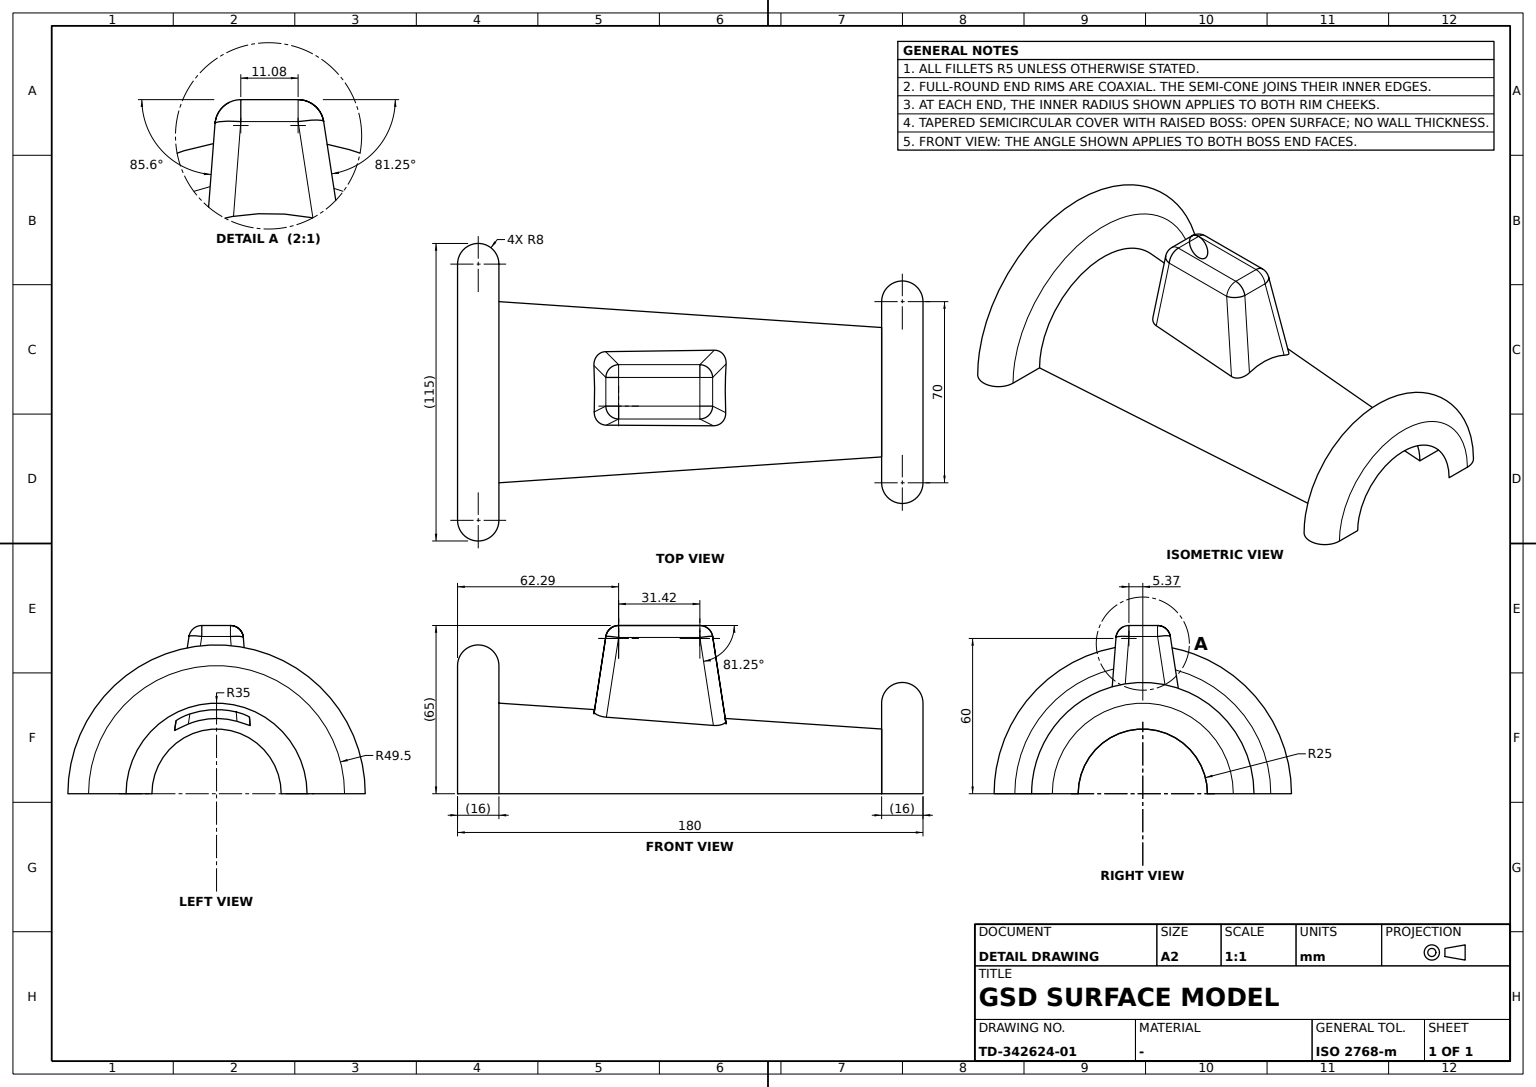
ISO-10303-21;
HEADER;
FILE_DESCRIPTION((''),'2;1');
FILE_NAME('','',(''),(''),'','','');
FILE_SCHEMA(('AUTOMOTIVE_DESIGN'));
ENDSEC;
DATA;
#1=CIRCLE('',#302,4.999999999999998224);
#2=VERTEX_POINT('',#358);
#3=DIRECTION('',(1.000000000000000000,0.000000000000000000,0.000000000000000000));
#4=DIRECTION('',(0.1516196087203265097,0.07580980435783682414,0.9855274566518792412));
#5=CARTESIAN_POINT('',(82.88880034649218942,16.11741507233864823,25.23680202979879894));
#6=PRODUCT_DEFINITION('','',#656,#165);
#7=ORIENTED_EDGE('',*,*,#105,.T.);
#8=DIRECTION('',(1.000000000000000000,1.487698852997710001E-15,0.000000000000000000));
#9=ORIENTED_EDGE('',*,*,#105,.F.);
#10=VECTOR('',#469,1000.000000000000114);
#11=ADVANCED_FACE('',(#30),#593,.F.);
#13=CARTESIAN_POINT('',(54.28959478410899919,0.1702804562384080123,65.00000000000000000));
#14=CARTESIAN_POINT('',(95.49929889487789580,-0.1677061014116459914,29.25455718508739622));
#15=AXIS2_PLACEMENT_3D('',#572,#347,#4);
#16=ADVANCED_FACE('',(#351),#800,.T.);
#17=DIRECTION('',(0.000000000000000000,0.000000000000000000,1.000000000000000000));
#18=CARTESIAN_POINT('',(156.0000000148439767,0.000000000000000000,0.000000000000000000));
#19=PLANE('',#403);
#20=DIRECTION('',(-0.1516196087154709493,0.07580980438481749184,0.9855274566505506373));
#21=CARTESIAN_POINT('',(47.47618292701569942,-12.26897543147416059,29.91601842641244957));
#23=DIRECTION('',(1.000000000000000000,0.000000000000000000,0.000000000000000000));
#24=ORIENTED_EDGE('',*,*,#110,.T.);
#25=AXIS2_PLACEMENT_3D('',#18,#337,#721);
#27=SPHERICAL_SURFACE('',#463,5.000000000000000000);
#28=VECTOR('',#773,1000.000000000000000);
#29=EDGE_CURVE('',#776,#556,#68,.T.);
#30=FACE_OUTER_BOUND('',#231,.T.);
#31=APPLICATION_CONTEXT('configuration controlled 3d designs of mechanical parts and assemblies');
#34=DIRECTION('',(0.000000000000000000,1.000000000000000000,0.000000000000000000));
#35=DIRECTION('',(1.000000000000000000,0.000000000000000000,0.000000000000000000));
#36=CARTESIAN_POINT('',(0.000000000000000000,49.50000000000000000,0.000000000000000000));
#37=CARTESIAN_POINT('',(93.17356924397489593,-6.630497073329739699,44.37179991595679951));
#38=ORIENTED_EDGE('',*,*,#428,.F.);
#39=EDGE_CURVE('',#755,#832,#545,.T.);
#40=FACE_OUTER_BOUND('',#717,.T.);
#41=LINE('',#300,#575);
#42=ORIENTED_EDGE('',*,*,#29,.F.);
#43=DIRECTION('',(0.000000000000000000,-1.000000000000000000,0.000000000000000000));
#44=EDGE_CURVE('',#748,#581,#379,.T.);
#45=TOROIDAL_SURFACE('',#640,49.50000000000000000,8.000000000000000000);
#46=EDGE_LOOP('',(#705,#697,#655,#76));
#47=AXIS2_PLACEMENT_3D('',#732,#421,#443);
#48=DIRECTION('',(0.1516196087157820060,-0.07580980435789032301,-0.9855274566525742408));
#49=VERTEX_POINT('',#150);
#50=DIRECTION('',(0.000000000000000000,1.000000000000000000,0.000000000000000000));
#51=DIRECTION('',(-0.9883716976506171648,-1.387778780781446267E-15,0.1520571842539412133));
#52=AXIS2_PLACEMENT_3D('',#486,#93,#548);
#53=ADVANCED_FACE('',(#412),#668,.F.);
#54=ORIENTED_EDGE('',*,*,#362,.F.);
#55=CARTESIAN_POINT('',(44.99136965415389255,-3.305473042556384744,32.44390275020669634));
#56=CARTESIAN_POINT('',(90.65226370469589767,-5.369844303690290310,60.76028592126970551));
#57=DIRECTION('',(0.000000000000000000,-1.000000000000000000,0.000000000000000000));
#58=AXIS2_PLACEMENT_3D('',#564,#439,#174);
#59=EDGE_CURVE('',#70,#810,#621,.T.);
#60=EDGE_LOOP('',(#464,#339,#440,#141));
#61=CARTESIAN_POINT('',(49.34773629585589561,5.710405216167110609,60.76028592126970551));
#62=DIRECTION('',(0.000000000000000000,-0.9970544855015814889,0.07669649888473735466));
#63=LINE('',#623,#397);
#64=ORIENTED_EDGE('',*,*,#588,.T.);
#65=CARTESIAN_POINT('',(49.34773629585589561,-5.369844303690300080,60.76028592126970551));
#66=CARTESIAN_POINT('',(172.0000000002759748,35.00000000590325300,0.000000000000000000));
#67=LINE('',#37,#113);
#68=CIRCLE('',#524,49.50000000000000000);
#69=VECTOR('',#192,1000.000000000000000);
#70=VERTEX_POINT('',#763);
#71=CARTESIAN_POINT('',(93.16960352932520095,-12.47231050528696095,26.45346037570174857));
#72=PLANE('',#615);
#74=CARTESIAN_POINT('',(172.0000000002759748,0.000000000000000000,0.000000000000000000));
#76=ORIENTED_EDGE('',*,*,#307,.F.);
#77=CARTESIAN_POINT('',(172.0000000002759748,25.00000000000000000,0.000000000000000000));
#78=VERTEX_POINT('',#366);
#80=CARTESIAN_POINT('',(48.38591088909750226,15.58465777130594887,28.25883129024764884));
#81=CARTESIAN_POINT('',(82.00000000742190309,29.99999999704840192,7.347880794161179401E-15));
#82=DIRECTION('',(0.1516196087157820060,-0.07580980435789032301,-0.9855274566525742408));
#83=CARTESIAN_POINT('',(54.28959478410899919,10.65226370442009873,60.76028592126970551));
#84=DIRECTION('',(0.000000000000000000,1.000000000000000000,0.000000000000000000));
#85=DIRECTION('',(-3.157196726277788912E-16,-0.9883716976506172758,-0.1520571842539405194));
#86=CARTESIAN_POINT('',(95.00000000027590374,1.250000000000000000,32.50000000000000000));
#87=CARTESIAN_POINT('',(46.67622673502380337,-11.78862029462323946,30.16918636838424916));
#88=CARTESIAN_POINT('',(85.71040521644290777,5.710405216167009357,65.00000000000000000));
#89=DIRECTION('',(1.000000000000000000,0.000000000000000000,0.000000000000000000));
#90=VERTEX_POINT('',#831);
#91=EDGE_LOOP('',(#491,#214,#452));
#93=DIRECTION('',(0.000000000000000000,0.000000000000000000,1.000000000000000000));
#94=B_SPLINE_CURVE_WITH_KNOTS('',5,(#199,#371,#688,#647,#388,#681),.UNSPECIFIED.,.F.,.F.,(6,6),(18.38578600851790057,77.10356617724089290),.UNSPECIFIED.);
#95=EDGE_CURVE('',#581,#176,#606,.T.);
#96=ORIENTED_EDGE('',*,*,#211,.T.);
#97=CIRCLE('',#311,4.999999999999999112);
#98=CARTESIAN_POINT('',(95.85588611873869525,10.91402763020971989,26.93674022999184814));
#99=AXIS2_PLACEMENT_3D('',#36,#489,#675);
#100=ADVANCED_FACE('',(#703),#684,.F.);
#101=VERTEX_POINT('',#490);
#103=DIRECTION('',(0.000000000000000000,1.000000000000000000,0.000000000000000000));
#104=CARTESIAN_POINT('',(88.50134585785460217,13.44320434583184110,42.61917175209315189));
#105=EDGE_CURVE('',#624,#827,#94,.T.);
#106=VERTEX_POINT('',#808);
#107=DIRECTION('',(-0.1516196087157805350,-0.07580980435789033689,-0.9855274566525744628));
#108=CARTESIAN_POINT('',(85.71040521644290777,1.624594337250419906,60.00000000000000000));
#109=CIRCLE('',#817,8.000000000000000000);
#110=EDGE_CURVE('',#810,#504,#63,.T.);
#111=ORIENTED_EDGE('',*,*,#805,.F.);
#112=LINE('',#557,#359);
#113=VECTOR('',#172,1000.000000000000000);
#114=AXIS2_PLACEMENT_3D('',#210,#607,#401);
#115=CARTESIAN_POINT('',(91.69480024177698851,16.22519456258525139,24.45135853039099771));
#116=ORIENTED_EDGE('',*,*,#812,.T.);
#117=DIRECTION('',(-1.798561299892755094E-15,1.000000000000000000,0.000000000000000000));
#119=EDGE_LOOP('',(#448,#733,#771,#200));
#120=CARTESIAN_POINT('',(49.34773629585589561,0.1702804562384055143,60.76028592126970551));
#121=DIRECTION('',(-0.1516196087157810068,-0.07580980435789033689,-0.9855274566525743518));
#122=EDGE_CURVE('',#660,#176,#322,.T.);
#123=ORIENTED_EDGE('',*,*,#247,.T.);
#124=CARTESIAN_POINT('',(164.0000000002760032,0.000000000000000000,0.000000000000000000));
#125=DIRECTION('',(1.000000000000000000,0.000000000000000000,0.000000000000000000));
#126=B_SPLINE_CURVE_WITH_KNOTS('',5,(#206,#5,#779,#518,#592,#411),.UNSPECIFIED.,.F.,.F.,(6,6),(7.118056443238479858,66.79193510323329974),.UNSPECIFIED.);
#127=VECTOR('',#57,1000.000000000000000);
#128=EDGE_CURVE('',#354,#755,#175,.T.);
#129=ORIENTED_EDGE('',*,*,#216,.T.);
#130=CARTESIAN_POINT('',(91.83171135900498427,-12.91060546447489976,26.34200180688025128));
#131=CARTESIAN_POINT('',(45.00000000027600322,1.250000000000000000,32.50000000000000000));
#132=ORIENTED_EDGE('',*,*,#281,.T.);
#133=EDGE_CURVE('',#2,#767,#234,.T.);
#134=DIRECTION('',(1.000000000000000000,0.000000000000000000,0.000000000000000000));
#136=CARTESIAN_POINT('',(95.05820376501719693,14.20966587805240167,25.41776108393125000));
#137=ORIENTED_EDGE('',*,*,#396,.T.);
#138=CARTESIAN_POINT('',(95.69487478325380891,-7.891149842969199746,27.98331391064385087));
#139=CARTESIAN_POINT('',(70.00000000027591796,15.00000000000000000,32.50000000000000000));
#140=DIRECTION('',(-1.000000000000000000,0.000000000000000000,0.000000000000000000));
#141=ORIENTED_EDGE('',*,*,#737,.F.);
#142=CARTESIAN_POINT('',(47.25216781269080002,15.16623239705239889,28.57288902478754977));
#144=EDGE_LOOP('',(#132,#244,#535,#190));
#145=DIRECTION('',(0.1503292056005669231,0.1503292056005649246,-0.9771398364036775197));
#146=EDGE_CURVE('',#570,#185,#552,.T.);
#147=DIRECTION('',(0.000000000000000000,1.000000000000000000,0.000000000000000000));
#148=CARTESIAN_POINT('',(48.97379723481959957,15.66647489519125003,28.16791318125715193));
#150=CARTESIAN_POINT('',(172.0000000002759748,35.00000000590325300,0.000000000000000000));
#151=CARTESIAN_POINT('',(45.25537269875960078,-9.950597534008000622,30.92943207874249723));
#153=DIRECTION('',(0.000000000000000000,0.000000000000000000,1.000000000000000000));
#154=CARTESIAN_POINT('',(95.69487478325380891,-7.891149842969199746,27.98331391064385087));
#155=AXIS2_PLACEMENT_3D('',#457,#89,#521);
#156=CARTESIAN_POINT('',(49.40154472305160027,-12.72446056995518049,29.58201259058274957));
#157=ADVANCED_FACE('',(#742),#512,.T.);
#159=CARTESIAN_POINT('',(164.0000000002760032,35.00000000575105474,0.000000000000000000));
#160=ORIENTED_EDGE('',*,*,#236,.T.);
#163=CARTESIAN_POINT('',(54.28959478410899919,5.710405216167009357,60.00000000000000000));
#164=CARTESIAN_POINT('',(95.60250083177299985,6.177536609898770514,28.58374459526904943));
#165=DESIGN_CONTEXT('detailed design',#292,'design');
#166=CARTESIAN_POINT('',(73.17931969364630618,-5.369844303690290310,60.00000000000000000));
#167=CIRCLE('',#820,35.00000000575105474);
#168=EDGE_CURVE('',#644,#748,#67,.T.);
#169=CARTESIAN_POINT('',(95.22242292336110836,13.93223856638788050,25.55853269397865191));
#170=DIRECTION('',(0.000000000000000000,1.000000000000000000,0.000000000000000000));
#171=EDGE_CURVE('',#422,#638,#41,.T.);
#172=DIRECTION('',(0.1516196087157820060,-0.07580980435789032301,-0.9855274566525742408));
#173=VERTEX_POINT('',#241);
#174=DIRECTION('',(-0.9883716976506171648,-1.387778780781446267E-15,0.1520571842539412133));
#175=LINE('',#627,#127);
#176=VERTEX_POINT('',#598);
#177=DIRECTION('',(0.9923906217041431610,-0.1231294195294709432,0.000000000000000000));
#178=CIRCLE('',#487,35.00000000575105474);
#179=TOROIDAL_SURFACE('',#540,35.00000000575105474,8.000000000000000000);
#180=ORIENTED_EDGE('',*,*,#595,.F.);
#181=DIRECTION('',(0.000000000000000000,-1.000000000000000000,0.000000000000000000));
#182=EDGE_CURVE('',#49,#708,#178,.T.);
#183=CYLINDRICAL_SURFACE('',#416,5.000000000000004441);
#184=CIRCLE('',#266,8.000000000000000000);
#185=VERTEX_POINT('',#471);
#186=VECTOR('',#43,1000.000000000000000);
#187=CARTESIAN_POINT('',(44.81399954011035192,8.945272495005509583,31.29099700892375324));
#188=CYLINDRICAL_SURFACE('',#754,5.000000000000000000);
#189=EDGE_CURVE('',#422,#348,#650,.T.);
#190=ORIENTED_EDGE('',*,*,#338,.F.);
#191=VECTOR('',#23,1000.000000000000000);
#192=DIRECTION('',(0.000000000000000000,1.000000000000000000,0.000000000000000000));
#193=FACE_OUTER_BOUND('',#455,.T.);
#194=DIRECTION('',(5.551115123125781913E-15,-1.000000000000000000,0.000000000000000000));
#195=EDGE_CURVE('',#297,#638,#591,.T.);
#196=ORIENTED_EDGE('',*,*,#493,.F.);
#197=LINE('',#120,#426);
#198=CARTESIAN_POINT('',(85.71040521644290777,-5.369844303690290310,65.00000000000000000));
#199=CARTESIAN_POINT('',(90.94180352461540906,-12.97081588528443952,26.37939349130229871));
#200=ORIENTED_EDGE('',*,*,#690,.T.);
#201=CARTESIAN_POINT('',(90.94180352461540906,-12.97081588528443952,26.37939349130229871));
#202=FACE_OUTER_BOUND('',#400,.T.);
#203=LINE('',#13,#342);
#204=VERTEX_POINT('',#770);
#205=DIRECTION('',(-0.1503292056053934789,-0.1503292056004535138,0.9771398364029521000));
#206=CARTESIAN_POINT('',(91.29228649926641026,16.23414498724360300,24.47805758291660183));
#207=AXIS2_PLACEMENT_3D('',#289,#407,#791);
#208=AXIS2_PLACEMENT_3D('',#563,#181,#651);
#209=VERTEX_POINT('',#77);
#210=CARTESIAN_POINT('',(87.86989544899509497,7.869895448719248954,45.96331348841030007));
#211=EDGE_CURVE('',#755,#767,#286,.T.);
#212=DIRECTION('',(-1.000000000000000000,0.000000000000000000,0.000000000000000000));
#214=ORIENTED_EDGE('',*,*,#281,.F.);
#216=EDGE_CURVE('',#660,#90,#97,.T.);
#217=FACE_BOUND('',#368,.T.);
#218=CARTESIAN_POINT('',(-8.000000000000000000,49.49999999984779464,0.000000000000000000));
#219=CARTESIAN_POINT('',(44.86237560386445011,-7.612524649686020162,31.60544142332520678));
#220=DIRECTION('',(0.000000000000000000,0.9883716976506171648,0.1520571842539412133));
#221=EDGE_CURVE('',#176,#297,#126,.T.);
#222=ORIENTED_EDGE('',*,*,#171,.F.);
#223=VECTOR('',#806,1000.000000000000000);
#224=CARTESIAN_POINT('',(48.49555997888629832,-12.63087847504785977,29.68878102991919832));
#226=DIRECTION('',(-1.000000000000000000,0.000000000000000000,-2.261376221629570055E-16));
#227=ORIENTED_EDGE('',*,*,#447,.F.);
#228=EDGE_CURVE('',#504,#348,#203,.T.);
#230=DIRECTION('',(-0.1503292056005659516,0.1503292056005649524,-0.9771398364036777417));
#231=EDGE_LOOP('',(#437,#404,#54,#796));
#232=SHAPE_DEFINITION_REPRESENTATION(#255,#823);
#233=CARTESIAN_POINT('',(172.0000000002759748,0.000000000000000000,0.000000000000000000));
#234=LINE('',#392,#539);
#235=DIRECTION('',(0.9931796065548538222,-0.1165944643777977463,0.000000000000000000));
#236=EDGE_CURVE('',#481,#348,#807,.T.);
#237=B_SPLINE_CURVE_WITH_KNOTS('',5,(#219,#473,#419,#724,#151,#414,#669,#87,#21,#792,#224,#477,#730,#156,#336),.UNSPECIFIED.,.F.,.F.,(6,3,3,3,6),(0.000000000000000000,3.367873996148655014,6.743899523194690993,10.08085567418961936,11.12778031997254047),.UNSPECIFIED.);
#238=CARTESIAN_POINT('',(92.14431663577398979,16.18187771320840085,24.44365995166524996));
#239=ORIENTED_EDGE('',*,*,#110,.F.);
#240=CARTESIAN_POINT('',(54.28959478410899919,-5.369844303690290310,60.00000000000000000));
#241=CARTESIAN_POINT('',(44.86237560386445011,-7.612524649686020162,31.60544142332520678));
#242=VERTEX_POINT('',#265);
#243=SPHERICAL_SURFACE('',#387,5.000000000000000000);
#244=ORIENTED_EDGE('',*,*,#493,.T.);
#245=DIRECTION('',(-0.9923906217041432720,0.1231294195294691390,0.000000000000000000));
#246=AXIS2_PLACEMENT_3D('',#781,#82,#533);
#247=EDGE_CURVE('',#101,#504,#578,.T.);
#248=ORIENTED_EDGE('',*,*,#122,.F.);
#249=CARTESIAN_POINT('',(92.28189212856520385,-12.80921589528385951,26.35774575813620046));
#250=LINE('',#503,#373);
#251=CIRCLE('',#441,4.999999999999997335);
#252=ORIENTED_EDGE('',*,*,#396,.F.);
#253=DIRECTION('',(1.000000000000000000,0.000000000000000000,0.000000000000000000));
#254=DIRECTION('',(-1.000000000000000000,-1.734723475976808080E-15,0.000000000000000000));
#255=PRODUCT_DEFINITION_SHAPE('','',#6);
#256=CARTESIAN_POINT('',(95.79170671442220453,12.40814064802130190,26.29498048308840197));
#257=EDGE_LOOP('',(#751,#672,#838,#384));
#258=FACE_OUTER_BOUND('',#619,.T.);
#259=CARTESIAN_POINT('',(82.00000000742190309,-29.99999999704840192,-3.673940397080589700E-15));
#260=AXIS2_PLACEMENT_3D('',#131,#296,#436);
#261=CARTESIAN_POINT('',(92.58565538170759623,16.08165661946335234,24.47417419825289642));
#262=EDGE_LOOP('',(#434,#764,#227));
#263=CARTESIAN_POINT('',(91.37388575645711342,-12.95788146452606071,26.35322200983669916));
#264=DIRECTION('',(0.000000000000000000,-1.224646799147353947E-16,-1.000000000000000000));
#265=CARTESIAN_POINT('',(172.0000000002759748,-25.00000000000000000,0.000000000000000000));
#266=AXIS2_PLACEMENT_3D('',#577,#264,#268);
#267=ORIENTED_EDGE('',*,*,#247,.F.);
#268=DIRECTION('',(0.000000000000000000,-1.000000000000000000,1.224646799147351482E-16));
#269=CARTESIAN_POINT('',(54.28959478410899919,5.710405216167009357,60.00000000000000000));
#270=ORIENTED_EDGE('',*,*,#122,.T.);
#271=ADVANCED_FACE('',(#784,#217),#328,.T.);
#272=CARTESIAN_POINT('',(48.67745418916620537,15.63802761698750210,28.20666023586069926));
#273=AXIS2_PLACEMENT_3D('',#108,#433,#766);
#274=ORIENTED_EDGE('',*,*,#304,.T.);
#276=B_SPLINE_CURVE_WITH_KNOTS('',5,(#445,#187,#499,#752,#381,#636,#55,#828,#505),.UNSPECIFIED.,.F.,.F.,(6,3,6),(7.868597663103630069,17.68701620253764872,32.60825157004950370),.UNSPECIFIED.);
#277=DIRECTION('',(-1.387778780781445478E-15,1.000000000000000000,0.000000000000000000));
#278=ORIENTED_EDGE('',*,*,#95,.T.);
#280=FACE_OUTER_BOUND('',#649,.T.);
#281=EDGE_CURVE('',#90,#565,#795,.T.);
#282=EDGE_LOOP('',(#301,#137,#712,#816));
#284=DIRECTION('',(-1.000000000000000000,0.000000000000000000,0.000000000000000000));
#285=AXIS2_PLACEMENT_3D('',#233,#483,#34);
#286=CIRCLE('',#25,24.99999999409675056);
#287=ORIENTED_EDGE('',*,*,#211,.F.);
#288=CARTESIAN_POINT('',(70.00000000027591796,5.710405216167009357,65.00000000000000000));
#289=CARTESIAN_POINT('',(8.000000000000000000,49.50000000000000000,0.000000000000000000));
#290=CIRCLE('',#626,35.00000000000000000);
#291=PLANE('',#52);
#292=APPLICATION_CONTEXT('configuration controlled 3d designs of mechanical parts and assemblies');
#293=DIRECTION('',(0.000000000000000000,1.000000000000000000,0.000000000000000000));
#294=ADVANCED_FACE('',(#571),#320,.F.);
#295=LINE('',#288,#191);
#296=DIRECTION('',(0.9883716976506171648,1.543903893619358314E-15,-0.1520571842539411855));
#297=VERTEX_POINT('',#760);
#299=LINE('',#830,#718);
#300=CARTESIAN_POINT('',(47.04604209059689879,8.012099421426050583,45.79927358708630436));
#301=ORIENTED_EDGE('',*,*,#747,.T.);
#302=AXIS2_PLACEMENT_3D('',#818,#107,#51);
#303=DIRECTION('',(-0.1503292056005664235,0.1503292056005649524,-0.9771398364036775197));
#304=EDGE_CURVE('',#90,#581,#833,.T.);
#305=EDGE_LOOP('',(#287,#444,#308,#549));
#306=DIRECTION('',(-0.1503292056005659516,0.1503292056005649524,-0.9771398364036777417));
#307=EDGE_CURVE('',#363,#422,#197,.T.);
#308=ORIENTED_EDGE('',*,*,#740,.T.);
#309=LINE('',#702,#399);
#310=DIRECTION('',(0.1231294195294691390,0.9923906217041432720,0.000000000000000000));
#311=AXIS2_PLACEMENT_3D('',#775,#145,#584);
#312=VECTOR('',#226,1000.000000000000000);
#313=ORIENTED_EDGE('',*,*,#195,.T.);
#314=ADVANCED_FACE('',(#258),#179,.T.);
#315=DIRECTION('',(-1.923808848762939692E-15,1.000000000000000000,-6.412696162543140194E-16));
#316=CARTESIAN_POINT('',(172.0000000002759748,-30.00000000295159808,0.000000000000000000));
#317=VECTOR('',#774,1000.000000000000000);
#318=CARTESIAN_POINT('',(95.85588611873869525,10.91402763020971989,26.93674022999184814));
#319=ORIENTED_EDGE('',*,*,#560,.F.);
#320=PLANE('',#778);
#321=EDGE_CURVE('',#185,#106,#438,.T.);
#322=LINE('',#104,#367);
#323=EDGE_LOOP('',(#693,#682,#612,#180));
#324=CIRCLE('',#365,4.999999999999998224);
#325=DIRECTION('',(0.1503292056005675337,0.1503292056005650357,-0.9771398364036772977));
#326=CARTESIAN_POINT('',(0.000000000000000000,0.000000000000000000,0.000000000000000000));
#327=CARTESIAN_POINT('',(94.23487094699301281,15.17431418557760026,24.91805486836235062));
#328=CONICAL_SURFACE('',#369,24.99999999409675056,0.06746502455486373673);
#329=ORIENTED_EDGE('',*,*,#44,.F.);
#330=CARTESIAN_POINT('',(93.69957373599699224,-12.13855933293189970,26.56878299509994790));
#331=CARTESIAN_POINT('',(156.0000000148439767,-24.99999999992395061,0.000000000000000000));
#332=DIRECTION('',(0.000000000000000000,0.000000000000000000,1.000000000000000000));
#334=EDGE_CURVE('',#832,#776,#509,.T.);
#335=ORIENTED_EDGE('',*,*,#189,.T.);
#336=CARTESIAN_POINT('',(49.54917917777090253,-12.72532453436723898,29.57078105322610284));
#337=DIRECTION('',(1.000000000000000000,0.000000000000000000,0.000000000000000000));
#338=EDGE_CURVE('',#90,#644,#309,.T.);
#339=ORIENTED_EDGE('',*,*,#171,.T.);
#341=CARTESIAN_POINT('',(44.74434788533795171,10.31379362668499944,30.83826125290294939));
#342=VECTOR('',#84,1000.000000000000000);
#343=CARTESIAN_POINT('',(95.56082365354178876,-3.992517549636114715,28.85464625377194992));
#345=LINE('',#357,#715);
#346=DIRECTION('',(0.000000000000000000,1.000000000000000000,0.000000000000000000));
#347=DIRECTION('',(-8.673617379884037013E-18,0.9970544855015815999,-0.07669649888473702160));
#348=VERTEX_POINT('',#631);
#349=LINE('',#423,#312);
#350=(LENGTH_UNIT()NAMED_UNIT(*)SI_UNIT(.MILLI.,.METRE.));
#351=FACE_OUTER_BOUND('',#376,.T.);
#353=CARTESIAN_POINT('',(54.28959478410899919,-5.369844303690290310,60.00000000000000000));
#354=VERTEX_POINT('',#377);
#355=VECTOR('',#325,1000.000000000000114);
#357=CARTESIAN_POINT('',(-8.000000000000000000,-42.24999999992390087,0.000000000000000000));
#358=CARTESIAN_POINT('',(156.0000000002760032,-35.00000000575105474,4.286263797720040190E-15));
#359=VECTOR('',#121,1000.000000000000114);
#360=DIRECTION('',(1.000000000000000000,0.000000000000000000,0.000000000000000000));
#361=DIRECTION('',(0.000000000000000000,-1.000000000000000000,0.000000000000000000));
#362=EDGE_CURVE('',#570,#78,#837,.T.);
#363=VERTEX_POINT('',#65);
#364=CYLINDRICAL_SURFACE('',#58,4.999999999999998224);
#365=AXIS2_PLACEMENT_3D('',#163,#230,#220);
#366=CARTESIAN_POINT('',(-8.000000000000000000,-49.50000000000000000,6.062001655779399300E-15));
#367=VECTOR('',#488,999.9999999999998863);
#368=EDGE_LOOP('',(#635,#508,#520,#459,#780,#329,#252,#7));
#369=AXIS2_PLACEMENT_3D('',#525,#140,#346);
#370=CARTESIAN_POINT('',(95.69487478325380891,-7.891149842969199746,27.98331391064385087));
#371=CARTESIAN_POINT('',(82.66400464164398443,-12.92098763422904106,27.02716075502254967));
#372=ORIENTED_EDGE('',*,*,#29,.T.);
#373=VECTOR('',#757,1000.000000000000114);
#374=CYLINDRICAL_SURFACE('',#825,5.000000000000002665);
#375=EDGE_CURVE('',#644,#810,#611,.T.);
#376=EDGE_LOOP('',(#663,#821,#372,#38));
#377=CARTESIAN_POINT('',(156.0000000002760032,35.00000000575105474,0.000000000000000000));
#378=CARTESIAN_POINT('',(51.78055219077580063,13.16130629775324223,44.45150906460419549));
#379=B_SPLINE_CURVE_WITH_KNOTS('',5,(#154,#720,#735,#343,#14,#786,#164,#723,#425),.UNSPECIFIED.,.F.,.F.,(6,3,6),(7.911103992056570000,17.48065422465330343,35.49133295374355157),.UNSPECIFIED.);
#380=EDGE_LOOP('',(#476,#759,#239,#196));
#381=CARTESIAN_POINT('',(45.00474972572950350,2.540943037684209926,32.53087321544789745));
#382=CARTESIAN_POINT('',(54.28959478410899919,-0.7472812842481779683,60.00000000000000000));
#384=ORIENTED_EDGE('',*,*,#304,.F.);
#385=CARTESIAN_POINT('',(92.58343921325520398,-12.71400336806163978,26.38140407509665053));
#386=CARTESIAN_POINT('',(0.000000000000000000,0.000000000000000000,0.000000000000000000));
#387=AXIS2_PLACEMENT_3D('',#496,#749,#177);
#388=CARTESIAN_POINT('',(57.82928910708479719,-12.77378016767503865,28.94085782022455078));
#389=ORIENTED_EDGE('',*,*,#680,.F.);
#390=CARTESIAN_POINT('',(93.25407491171729646,8.312216423188360181,43.84851307563079814));
#391=DIRECTION('',(1.000000000000000000,0.000000000000000000,0.000000000000000000));
#392=CARTESIAN_POINT('',(156.0000000148439767,-29.99999999992395061,0.000000000000000000));
#393=EDGE_LOOP('',(#116,#270,#574,#587));
#394=CARTESIAN_POINT('',(91.08570028369999250,-12.97168207281880115,26.36813305335579827));
#395=DIRECTION('',(1.000000000000000000,0.000000000000000000,0.000000000000000000));
#396=EDGE_CURVE('',#624,#748,#836,.T.);
#397=VECTOR('',#643,1000.000000000000000);
#398=DIRECTION('',(1.000000000000000000,0.000000000000000000,0.000000000000000000));
#399=VECTOR('',#449,1000.000000000000000);
#400=EDGE_LOOP('',(#42,#689,#495,#111));
#401=DIRECTION('',(0.9883716976506169427,3.469446951953614682E-16,0.1520571842539425733));
#402=CARTESIAN_POINT('',(45.08702962625869759,12.73369390222791964,29.90516772857334615));
#403=AXIS2_PLACEMENT_3D('',#139,#85,#205);
#404=ORIENTED_EDGE('',*,*,#485,.F.);
#405=CARTESIAN_POINT('',(49.27150959744269443,15.67034889108639995,28.14273220793869612));
#406=EDGE_CURVE('',#638,#173,#276,.T.);
#407=DIRECTION('',(1.000000000000000000,0.000000000000000000,0.000000000000000000));
#410=DIRECTION('',(0.000000000000000000,0.000000000000000000,1.000000000000000000));
#411=CARTESIAN_POINT('',(49.27150959744269443,15.67034889108639995,28.14273220793869612));
#412=FACE_OUTER_BOUND('',#257,.T.);
#414=CARTESIAN_POINT('',(45.73526101876370120,-10.75675299993679879,30.62000836728079989));
#415=DIRECTION('',(-0.1165944643777977463,-0.9931796065548538222,0.000000000000000000));
#416=AXIS2_PLACEMENT_3D('',#382,#699,#686);
#417=(NAMED_UNIT(*)SI_UNIT($,.STERADIAN.)SOLID_ANGLE_UNIT());
#418=ORIENTED_EDGE('',*,*,#541,.F.);
#419=CARTESIAN_POINT('',(44.88117671146429899,-8.573922403696609962,31.36289362578479611));
#421=DIRECTION('',(0.000000000000000000,-1.224646799147351975E-16,-1.000000000000000000));
#422=VERTEX_POINT('',#61);
#423=CARTESIAN_POINT('',(70.00000000027591796,-10.35511673119819953,60.38348249442369564));
#424=ADVANCED_FACE('',(#536),#594,.T.);
#425=CARTESIAN_POINT('',(95.85588611873869525,10.91402763020971989,26.93674022999184814));
#426=VECTOR('',#315,1000.000000000000000);
#427=FACE_OUTER_BOUND('',#380,.T.);
#428=EDGE_CURVE('',#204,#556,#787,.T.);
#429=CARTESIAN_POINT('',(92.88588346967999598,15.98306508511420176,24.51476435578769753));
#431=LINE('',#316,#186);
#432=AXIS2_PLACEMENT_3D('',#166,#360,#17);
#433=DIRECTION('',(0.000000000000000000,-1.000000000000000000,0.000000000000000000));
#434=ORIENTED_EDGE('',*,*,#375,.T.);
#435=CARTESIAN_POINT('',(51.37931008353369577,8.620689916742309222,41.08314944626044252));
#436=DIRECTION('',(0.1503292056005779420,-0.1503292056000529453,0.9771398364037545692));
#437=ORIENTED_EDGE('',*,*,#321,.T.);
#438=CIRCLE('',#498,35.00000000000000000);
#439=DIRECTION('',(-0.1516196087157805350,-0.07580980435789033689,-0.9855274566525744628));
#440=ORIENTED_EDGE('',*,*,#406,.T.);
#441=AXIS2_PLACEMENT_3D('',#240,#117,#254);
#442=CARTESIAN_POINT('',(156.0000000148439767,24.99999999992395061,0.000000000000000000));
#443=DIRECTION('',(0.000000000000000000,-1.000000000000000000,1.224646799147351482E-16));
#444=ORIENTED_EDGE('',*,*,#39,.T.);
#445=CARTESIAN_POINT('',(44.74434788533795171,10.31379362668499944,30.83826125290294939));
#446=LINE('',#378,#517);
#447=EDGE_CURVE('',#644,#70,#676,.T.);
#448=ORIENTED_EDGE('',*,*,#737,.T.);
#449=DIRECTION('',(1.282539232508642041E-15,-1.000000000000000000,6.412696162543210205E-16));
#450=CARTESIAN_POINT('',(93.99091676102828785,15.37597639342695111,24.81309271532975202));
#452=ORIENTED_EDGE('',*,*,#216,.F.);
#453=CARTESIAN_POINT('',(94.41830095388701238,-11.52617429664520010,26.78904607965900198));
#454=CARTESIAN_POINT('',(95.58182904051409423,13.19749207211669884,25.92405371302374917));
#455=EDGE_LOOP('',(#585,#532,#9,#484));
#456=CARTESIAN_POINT('',(95.59508661542660946,-9.322497419173259914,27.55319516760900100));
#457=CARTESIAN_POINT('',(85.71040521644290777,5.710405216167009357,60.00000000000000000));
#458=CARTESIAN_POINT('',(85.71040521644290777,5.710405216167000475,60.00000000000000000));
#459=ORIENTED_EDGE('',*,*,#221,.F.);
#460=EDGE_CURVE('',#173,#827,#237,.T.);
#461=CARTESIAN_POINT('',(8.000000000000000000,35.00000000000000000,8.572527594031479303E-15));
#462=DIRECTION('',(0.000000000000000000,1.000000000000000000,0.000000000000000000));
#463=AXIS2_PLACEMENT_3D('',#602,#235,#415);
#464=ORIENTED_EDGE('',*,*,#307,.T.);
#466=CARTESIAN_POINT('',(47.79671608356450463,15.42381999413469984,28.39278183557355106));
#467=ADVANCED_FACE('',(#427),#291,.T.);
#468=CIRCLE('',#155,5.000000000000004441);
#469=DIRECTION('',(-0.9977250982841701088,0.06741385802520860615,1.651163308974915055E-17));
#471=CARTESIAN_POINT('',(-8.000000000000000000,35.00000000000000000,0.000000000000000000));
#472=DIRECTION('',(1.000000000000000000,0.000000000000000000,0.000000000000000000));
#473=CARTESIAN_POINT('',(44.84473329274005238,-8.093719457027210851,31.49076640101704783));
#474=CYLINDRICAL_SURFACE('',#659,5.000000000000004441);
#475=CIRCLE('',#99,8.000000000000000000);
#476=ORIENTED_EDGE('',*,*,#550,.F.);
#477=CARTESIAN_POINT('',(49.10720282176270501,-12.70574662273625854,29.61170829729055143));
#479=CARTESIAN_POINT('',(-8.000000000000000000,49.50000000000000000,0.000000000000000000));
#480=AXIS2_PLACEMENT_3D('',#386,#642,#510);
#481=VERTEX_POINT('',#83);
#482=ADVANCED_FACE('',(#551),#734,.T.);
#483=DIRECTION('',(1.000000000000000000,0.000000000000000000,0.000000000000000000));
#484=ORIENTED_EDGE('',*,*,#747,.F.);
#485=EDGE_CURVE('',#78,#106,#345,.T.);
#486=CARTESIAN_POINT('',(0.000000000000000000,0.000000000000000000,65.00000000000000000));
#487=AXIS2_PLACEMENT_3D('',#74,#398,#654);
#488=DIRECTION('',(0.1503292056005664235,0.1503292056005649524,-0.9771398364036775197));
#489=DIRECTION('',(0.000000000000000000,0.000000000000000000,1.000000000000000000));
#490=CARTESIAN_POINT('',(54.28959478410899919,-10.35511673119819953,60.38348249442369564));
#491=ORIENTED_EDGE('',*,*,#801,.T.);
#492=LINE('',#695,#741);
#493=EDGE_CURVE('',#565,#810,#799,.T.);
#494=CARTESIAN_POINT('',(95.88745818558579970,11.41484323879720186,26.73152179548450036));
#495=ORIENTED_EDGE('',*,*,#362,.T.);
#496=CARTESIAN_POINT('',(85.71040521644280830,5.710405216167009357,60.00000000000000000));
#497=ORIENTED_EDGE('',*,*,#128,.T.);
#498=AXIS2_PLACEMENT_3D('',#567,#3,#698);
#499=CARTESIAN_POINT('',(44.87212247386959518,7.551452396107960041,31.66879607835879895));
#500=ORIENTED_EDGE('',*,*,#513,.F.);
#502=CARTESIAN_POINT('',(93.94955390235828929,-11.94891878325591961,26.63644170156274882));
#503=CARTESIAN_POINT('',(88.32610437052909447,-11.66296630824132130,43.38143799286299895));
#504=VERTEX_POINT('',#665);
#505=CARTESIAN_POINT('',(44.86237560386445011,-7.612524649686020162,31.60544142332520678));
#506=DIRECTION('',(0.000000000000000000,1.000000000000000000,0.000000000000000000));
#507=CARTESIAN_POINT('',(94.69267050433479938,14.72280005499678168,25.15354688604960032));
#508=ORIENTED_EDGE('',*,*,#406,.F.);
#509=LINE('',#839,#69);
#510=DIRECTION('',(1.000000000000000000,0.000000000000000000,0.000000000000000000));
#511=AXIS2_PLACEMENT_3D('',#569,#738,#194);
#512=CYLINDRICAL_SURFACE('',#273,5.000000000000004441);
#513=EDGE_CURVE('',#354,#2,#167,.T.);
#514=ORIENTED_EDGE('',*,*,#133,.F.);
#515=DIRECTION('',(0.000000000000000000,1.000000000000000000,0.000000000000000000));
#516=APPLICATION_PROTOCOL_DEFINITION('international standard','config_control_design',1994,#31);
#517=VECTOR('',#303,999.9999999999998863);
#518=CARTESIAN_POINT('',(66.08327803664619182,15.89057051478410010,26.71129165390364690));
#519=ADVANCED_FACE('',(#788),#27,.T.);
#520=ORIENTED_EDGE('',*,*,#195,.F.);
#521=DIRECTION('',(0.000000000000000000,0.000000000000000000,1.000000000000000000));
#522=CARTESIAN_POINT('',(54.28959478410899919,5.710405216167110609,60.00000000000000000));
#523=ORIENTED_EDGE('',*,*,#59,.T.);
#524=AXIS2_PLACEMENT_3D('',#728,#35,#293);
#525=CARTESIAN_POINT('',(156.0000000148439767,0.000000000000000000,0.000000000000000000));
#526=AXIS2_PLACEMENT_3D('',#353,#534,#614);
#527=ORIENTED_EDGE('',*,*,#236,.F.);
#528=CARTESIAN_POINT('',(8.000000000000000000,-42.25000000000000000,0.000000000000000000));
#530=EDGE_CURVE('',#776,#570,#475,.T.);
#531=CARTESIAN_POINT('',(54.28959478410899919,-5.369844303690290310,60.00000000000000000));
#532=ORIENTED_EDGE('',*,*,#704,.T.);
#533=DIRECTION('',(0.000000000000000000,-0.9970544855015814889,0.07669649888473735466));
#534=DIRECTION('',(-0.1186233085285600952,-0.9929393287979574323,0.000000000000000000));
#535=ORIENTED_EDGE('',*,*,#375,.F.);
#536=FACE_OUTER_BOUND('',#677,.T.);
#538=CARTESIAN_POINT('',(90.94180352461540906,-12.97081588528443952,26.37939349130229871));
#539=VECTOR('',#573,1000.000000000000000);
#540=AXIS2_PLACEMENT_3D('',#124,#646,#576);
#541=EDGE_CURVE('',#70,#101,#349,.T.);
#542=EDGE_LOOP('',(#814,#313,#222,#630));
#543=DIRECTION('',(1.000000000000000000,0.000000000000000000,0.000000000000000000));
#544=AXIS2_PLACEMENT_3D('',#568,#245,#310);
#545=LINE('',#81,#10);
#548=DIRECTION('',(1.000000000000000000,0.000000000000000000,0.000000000000000000));
#549=ORIENTED_EDGE('',*,*,#785,.F.);
#550=EDGE_CURVE('',#348,#565,#295,.T.);
#551=FACE_OUTER_BOUND('',#743,.T.);
#552=LINE('',#835,#634);
#553=EDGE_LOOP('',(#523,#24,#267,#418));
#554=CARTESIAN_POINT('',(172.0000000002759748,-35.00000000590325300,0.000000000000000000));
#555=DIRECTION('',(-0.1503292056005664512,0.1503292056005634814,-0.9771398364036778528));
#556=VERTEX_POINT('',#739);
#557=CARTESIAN_POINT('',(47.10505594986019418,-6.491184476688159677,46.18286367229750056));
#558=ORIENTED_EDGE('',*,*,#812,.F.);
#559=FACE_OUTER_BOUND('',#46,.T.);
#560=EDGE_CURVE('',#422,#481,#324,.T.);
#561=ORIENTED_EDGE('',*,*,#639,.F.);
#562=AXIS2_PLACEMENT_3D('',#458,#711,#694);
#563=CARTESIAN_POINT('',(85.71040521644290777,-5.369844303690290310,60.00000000000000000));
#564=CARTESIAN_POINT('',(52.51801325891039340,-6.255635066289579882,48.48472008620920093));
#565=VERTEX_POINT('',#88);
#567=CARTESIAN_POINT('',(-8.000000000000000000,0.000000000000000000,0.000000000000000000));
#568=CARTESIAN_POINT('',(54.28959478410899919,5.710405216167009357,60.00000000000000000));
#569=CARTESIAN_POINT('',(85.71040521644280830,-5.369844303690290310,60.00000000000000000));
#570=VERTEX_POINT('',#479);
#571=FACE_OUTER_BOUND('',#701,.T.);
#572=CARTESIAN_POINT('',(70.00000000027600322,-12.50000000000000000,32.50000000000000000));
#573=DIRECTION('',(0.000000000000000000,1.000000000000000000,0.000000000000000000));
#574=ORIENTED_EDGE('',*,*,#221,.T.);
#575=VECTOR('',#555,999.9999999999998863);
#576=DIRECTION('',(0.000000000000000000,1.000000000000000000,0.000000000000000000));
#577=CARTESIAN_POINT('',(0.000000000000000000,-49.50000000000000000,6.062001655779399300E-15));
#578=CIRCLE('',#750,5.000000000000004441);
#580=CARTESIAN_POINT('',(45.54283804013620340,13.57828883290601851,29.49263682702174805));
#581=VERTEX_POINT('',#98);
#582=CARTESIAN_POINT('',(95.68277507038769158,-8.849998887812729365,27.70267582980079979));
#583=LINE('',#259,#782);
#584=DIRECTION('',(0.9883716976506169427,3.469446951953614682E-16,0.1520571842539425733));
#585=ORIENTED_EDGE('',*,*,#541,.T.);
#586=CARTESIAN_POINT('',(46.34320931016520007,14.55101759307569864,28.96276863906010135));
#587=ORIENTED_EDGE('',*,*,#670,.F.);
#588=EDGE_CURVE('',#49,#354,#109,.T.);
#590=AXIS2_PLACEMENT_3D('',#522,#462,#332);
#591=B_SPLINE_CURVE_WITH_KNOTS('',5,(#405,#148,#272,#80,#466,#142,#657,#586,#666,#580,#402,#719,#661,#716,#341),.UNSPECIFIED.,.F.,.F.,(6,3,3,3,6),(-11.51261100740009979,-9.399964157141880605,-7.124267262507499865,-3.578268050059350003,0.000000000000000000),.UNSPECIFIED.);
#592=CARTESIAN_POINT('',(57.67887092382349579,15.77975038338809810,27.43162250797765012));
#593=PLANE('',#622);
#594=CYLINDRICAL_SURFACE('',#114,4.999999999999999112);
#595=EDGE_CURVE('',#209,#242,#648,.T.);
#597=FACE_OUTER_BOUND('',#553,.T.);
#598=CARTESIAN_POINT('',(91.29228649926641026,16.23414498724360300,24.47805758291660183));
#599=(NAMED_UNIT(*)PLANE_ANGLE_UNIT()SI_UNIT($,.RADIAN.));
#600=DIRECTION('',(-0.9883716976506169427,-5.273559366969494553E-16,-0.1520571842539426288));
#602=CARTESIAN_POINT('',(85.71040521644280830,-5.369844303690290310,60.00000000000000000));
#603=ADVANCED_FACE('',(#597),#736,.T.);
#604=FACE_OUTER_BOUND('',#323,.T.);
#605=ORIENTED_EDGE('',*,*,#550,.T.);
#606=B_SPLINE_CURVE_WITH_KNOTS('',5,(#318,#494,#707,#256,#454,#169,#136,#507,#327,#450,#804,#429,#261,#238,#115,#618,#813,#745),.UNSPECIFIED.,.F.,.F.,(6,3,3,3,3,6),(0.000000000000000000,3.895609381382159508,6.402614889156458489,8.760262675822469092,10.99985114066713976,11.95079642302754053),.UNSPECIFIED.);
#607=DIRECTION('',(0.1503292056005669231,0.1503292056005649246,-0.9771398364036775197));
#609=CARTESIAN_POINT('',(156.0000000002760032,0.000000000000000000,0.000000000000000000));
#610=ADVANCED_FACE('',(#280),#474,.T.);
#611=CIRCLE('',#208,5.000000000000004441);
#612=ORIENTED_EDGE('',*,*,#658,.F.);
#614=DIRECTION('',(-0.9929393287979574323,0.1186233085285600813,0.000000000000000000));
#615=AXIS2_PLACEMENT_3D('',#66,#391,#667);
#616=ORIENTED_EDGE('',*,*,#513,.T.);
#617=DIRECTION('',(0.000000000000000000,1.000000000000000000,0.000000000000000000));
#618=CARTESIAN_POINT('',(91.56048664960850658,16.23306953505460015,24.45702256365240146));
#619=EDGE_LOOP('',(#674,#64,#616,#561));
#620=CARTESIAN_POINT('',(156.0000000148439767,24.99999999992395061,0.000000000000000000));
#621=CIRCLE('',#511,5.000000000000000888);
#622=AXIS2_PLACEMENT_3D('',#218,#472,#147);
#623=CARTESIAN_POINT('',(70.00000000027591796,-5.369844303690290310,65.00000000000000000));
#624=VERTEX_POINT('',#538);
#625=FACE_OUTER_BOUND('',#91,.T.);
#626=AXIS2_PLACEMENT_3D('',#824,#125,#170);
#627=CARTESIAN_POINT('',(156.0000000148439767,29.99999999992395061,0.000000000000000000));
#628=ORIENTED_EDGE('',*,*,#690,.F.);
#629=CARTESIAN_POINT('',(88.18801494197700208,-6.608649166457330359,43.89553678402845094));
#630=ORIENTED_EDGE('',*,*,#560,.T.);
#631=CARTESIAN_POINT('',(54.28959478410899919,5.710405216167110609,65.00000000000000000));
#632=CARTESIAN_POINT('',(85.71040521644280830,10.65226370442009873,60.76028592126970551));
#633=PRODUCT_RELATED_PRODUCT_CATEGORY('','',(#645));
#634=VECTOR('',#361,1000.000000000000000);
#635=ORIENTED_EDGE('',*,*,#460,.F.);
#636=CARTESIAN_POINT('',(45.01408747448080305,-1.107195335485763987,32.59156858233155418));
#637=SPHERICAL_SURFACE('',#544,5.000000000000000000);
#638=VERTEX_POINT('',#794);
#639=EDGE_CURVE('',#708,#2,#815,.T.);
#640=AXIS2_PLACEMENT_3D('',#326,#395,#671);
#641=CARTESIAN_POINT('',(94.80446660762359556,-11.03692672447824030,26.96540847307355193));
#642=DIRECTION('',(0.000000000000000000,0.000000000000000000,1.000000000000000000));
#643=DIRECTION('',(-1.000000000000000000,0.000000000000000000,0.000000000000000000));
#644=VERTEX_POINT('',#56);
#645=PRODUCT('','','',(#761));
#646=DIRECTION('',(1.000000000000000000,0.000000000000000000,0.000000000000000000));
#647=CARTESIAN_POINT('',(66.10861073196069526,-12.82252091711287889,28.30722807753275205));
#648=CIRCLE('',#285,25.00000000000000000);
#649=EDGE_LOOP('',(#160,#605,#685,#558));
#650=CIRCLE('',#590,5.000000000000004441);
#651=DIRECTION('',(0.000000000000000000,0.000000000000000000,1.000000000000000000));
#652=DIRECTION('',(-0.9977250982841701088,-0.06741385802520860615,-8.255816544874579899E-18));
#653=AXIS2_PLACEMENT_3D('',#768,#253,#50);
#654=DIRECTION('',(0.000000000000000000,1.000000000000000000,0.000000000000000000));
#655=ORIENTED_EDGE('',*,*,#189,.F.);
#656=PRODUCT_DEFINITION_FORMATION_WITH_SPECIFIED_SOURCE('','',#645,.NOT_KNOWN.);
#657=CARTESIAN_POINT('',(46.98469307462670486,15.00861416487254907,28.67672561769210304));
#658=EDGE_CURVE('',#242,#708,#431,.T.);
#659=AXIS2_PLACEMENT_3D('',#726,#284,#153);
#660=VERTEX_POINT('',#632);
#661=CARTESIAN_POINT('',(44.74676542408794688,11.30947644330271906,30.49389888522365055));
#662=ADVANCED_FACE('',(#753),#188,.T.);
#663=ORIENTED_EDGE('',*,*,#740,.F.);
#665=CARTESIAN_POINT('',(54.28959478410899919,-5.369844303690290310,65.00000000000000000));
#666=CARTESIAN_POINT('',(45.81713236756800001,13.96963656865565895,29.28780423397259725));
#667=DIRECTION('',(0.000000000000000000,1.000000000000000000,0.000000000000000000));
#668=PLANE('',#819);
#669=CARTESIAN_POINT('',(46.02187066685019801,-11.12823878877212103,30.46540083422050316));
#670=EDGE_CURVE('',#481,#297,#446,.T.);
#671=DIRECTION('',(0.000000000000000000,1.000000000000000000,0.000000000000000000));
#672=ORIENTED_EDGE('',*,*,#168,.T.);
#673=ADVANCED_FACE('',(#559),#183,.T.);
#674=ORIENTED_EDGE('',*,*,#182,.F.);
#675=DIRECTION('',(0.000000000000000000,1.000000000000000000,0.000000000000000000));
#676=CIRCLE('',#246,5.000000000000002665);
#677=EDGE_LOOP('',(#274,#278,#248,#129));
#678=DIRECTION('',(0.000000000000000000,1.000000000000000000,0.000000000000000000));
#680=EDGE_CURVE('',#363,#504,#251,.T.);
#681=CARTESIAN_POINT('',(49.54917917777090253,-12.72532453436723898,29.57078105322610284));
#682=ORIENTED_EDGE('',*,*,#182,.T.);
#683=DIRECTION('',(-0.1516196087157805350,-0.07580980435789023975,-0.9855274566525744628));
#684=PLANE('',#260);
#685=ORIENTED_EDGE('',*,*,#801,.F.);
#686=DIRECTION('',(0.000000000000000000,0.000000000000000000,1.000000000000000000));
#687=AXIS2_PLACEMENT_3D('',#269,#8,#277);
#688=CARTESIAN_POINT('',(74.38625203040869849,-12.87157357124581836,27.66954357380460294));
#689=ORIENTED_EDGE('',*,*,#530,.T.);
#690=EDGE_CURVE('',#101,#363,#1,.T.);
#691=FACE_OUTER_BOUND('',#282,.T.);
#693=ORIENTED_EDGE('',*,*,#722,.T.);
#694=DIRECTION('',(0.000000000000000000,0.000000000000000000,1.000000000000000000));
#695=CARTESIAN_POINT('',(172.0000000002759748,30.00000000295159808,0.000000000000000000));
#697=ORIENTED_EDGE('',*,*,#228,.T.);
#698=DIRECTION('',(0.000000000000000000,1.000000000000000000,0.000000000000000000));
#699=DIRECTION('',(0.000000000000000000,-1.000000000000000000,0.000000000000000000));
#700=ADVANCED_FACE('',(#40),#637,.T.);
#701=EDGE_LOOP('',(#500,#497,#96,#514));
#702=CARTESIAN_POINT('',(90.65226370469589767,0.1702804562383554987,60.76028592126970551));
#703=FACE_OUTER_BOUND('',#60,.T.);
#704=EDGE_CURVE('',#101,#827,#299,.T.);
#705=ORIENTED_EDGE('',*,*,#680,.T.);
#706=CARTESIAN_POINT('',(95.36014488896290686,-10.07909845364516066,27.30256729004129923));
#707=CARTESIAN_POINT('',(95.86604913116050852,11.91498878678370055,26.51684424785144856));
#708=VERTEX_POINT('',#554);
#709=CARTESIAN_POINT('',(95.71589701281519069,-8.370480079848780619,27.84666941849344823));
#710=LINE('',#834,#317);
#711=DIRECTION('',(0.000000000000000000,-1.000000000000000000,0.000000000000000000));
#712=ORIENTED_EDGE('',*,*,#168,.F.);
#713=OPEN_SHELL('NONE',(#294,#314,#271,#777,#16,#729,#100,#662,#829,#424,#53,#762,#789,#772,#482,#673,#700,#610,#758,#157,#519,#603,#11,#467));
#714=CARTESIAN_POINT('',(8.000000000000000000,49.50000000000000000,0.000000000000000000));
#715=VECTOR('',#617,1000.000000000000000);
#716=CARTESIAN_POINT('',(44.71896381527650277,10.81254075261530012,30.67326479750450119));
#717=EDGE_LOOP('',(#335,#527,#319));
#718=VECTOR('',#683,1000.000000000000000);
#719=CARTESIAN_POINT('',(44.82685501559584651,11.79674540966505880,30.30261780816660178));
#720=CARTESIAN_POINT('',(95.63874433079689652,-6.611310042760990768,28.34816185161350077));
#721=DIRECTION('',(0.000000000000000000,1.000000000000000000,0.000000000000000000));
#722=EDGE_CURVE('',#209,#49,#492,.T.);
#723=CARTESIAN_POINT('',(95.70991817629649745,8.598592926010068638,27.88553185586630079));
#724=CARTESIAN_POINT('',(44.97137116200484996,-9.044380544065630190,31.22377704985575164));
#726=CARTESIAN_POINT('',(67.07665605273169263,5.710405216167009357,60.00000000000000000));
#727=PLANE('',#15);
#728=CARTESIAN_POINT('',(8.000000000000000000,0.000000000000000000,0.000000000000000000));
#729=ADVANCED_FACE('',(#744),#364,.T.);
#730=CARTESIAN_POINT('',(49.25411277022210044,-12.71794561250626110,29.59565989522785046));
#732=CARTESIAN_POINT('',(164.0000000002760032,-35.00000000575105474,4.286263797720040190E-15));
#733=ORIENTED_EDGE('',*,*,#460,.T.);
#734=SPHERICAL_SURFACE('',#526,5.000000000000000000);
#735=CARTESIAN_POINT('',(95.59396874879081452,-5.309832257771329722,28.63920313465330025));
#736=CYLINDRICAL_SURFACE('',#432,5.000000000000004441);
#737=EDGE_CURVE('',#363,#173,#112,.T.);
#738=DIRECTION('',(-1.000000000000000000,-5.684341886080810480E-15,0.000000000000000000));
#739=CARTESIAN_POINT('',(8.000000000000000000,-49.50000000000000000,0.000000000000000000));
#740=EDGE_CURVE('',#832,#204,#290,.T.);
#741=VECTOR('',#506,1000.000000000000000);
#742=FACE_OUTER_BOUND('',#144,.T.);
#743=EDGE_LOOP('',(#123,#389,#628));
#744=FACE_OUTER_BOUND('',#119,.T.);
#745=CARTESIAN_POINT('',(91.29228649926641026,16.23414498724360300,24.47805758291660183));
#746=SHELL_BASED_SURFACE_MODEL('',(#713));
#747=EDGE_CURVE('',#70,#624,#250,.T.);
#748=VERTEX_POINT('',#370);
#749=DIRECTION('',(0.1231294195294709432,0.9923906217041431610,-0.000000000000000000));
#750=AXIS2_PLACEMENT_3D('',#531,#212,#841);
#751=ORIENTED_EDGE('',*,*,#338,.T.);
#752=CARTESIAN_POINT('',(44.91841712245020091,6.137883524919519829,31.96971129413275037));
#753=FACE_OUTER_BOUND('',#542,.T.);
#754=AXIS2_PLACEMENT_3D('',#435,#306,#811);
#755=VERTEX_POINT('',#620);
#756=CARTESIAN_POINT('',(94.97805800414451483,-10.77428199321940028,27.05908024927644817));
#757=DIRECTION('',(0.1516196087157824779,-0.07580980435789022587,-0.9855274566525741298));
#758=ADVANCED_FACE('',(#625),#243,.T.);
#759=ORIENTED_EDGE('',*,*,#228,.F.);
#760=CARTESIAN_POINT('',(49.27150959744269443,15.67034889108639995,28.14273220793869612));
#761=MECHANICAL_CONTEXT('NONE',#31,'mechanical');
#762=ADVANCED_FACE('',(#691),#374,.T.);
#763=CARTESIAN_POINT('',(85.71040521644280830,-10.35511673119819953,60.38348249442369564));
#764=ORIENTED_EDGE('',*,*,#59,.F.);
#765=FACE_OUTER_BOUND('',#393,.T.);
#766=DIRECTION('',(0.000000000000000000,0.000000000000000000,1.000000000000000000));
#767=VERTEX_POINT('',#331);
#768=CARTESIAN_POINT('',(-8.000000000000000000,0.000000000000000000,0.000000000000000000));
#769=APPLICATION_PROTOCOL_DEFINITION('international standard','config_control_design',1994,#292);
#770=CARTESIAN_POINT('',(8.000000000000000000,-35.00000000000000000,-4.286263797015739652E-15));
#771=ORIENTED_EDGE('',*,*,#704,.F.);
#772=ADVANCED_FACE('',(#202),#45,.T.);
#773=DIRECTION('',(0.000000000000000000,-1.000000000000000000,0.000000000000000000));
#774=DIRECTION('',(1.000000000000000000,-3.392064332444355083E-16,2.261376221629570055E-16));
#775=CARTESIAN_POINT('',(85.71040521644280830,5.710405216167000475,60.00000000000000000));
#776=VERTEX_POINT('',#714);
#777=ADVANCED_FACE('',(#604),#72,.T.);
#778=AXIS2_PLACEMENT_3D('',#442,#134,#515);
#779=CARTESIAN_POINT('',(74.48479477967349283,16.00301356155105381,25.98041184991829766));
#780=ORIENTED_EDGE('',*,*,#95,.F.);
#781=CARTESIAN_POINT('',(85.71040521644280830,-5.369844303690290310,60.00000000000000000));
#782=VECTOR('',#652,1000.000000000000114);
#784=FACE_OUTER_BOUND('',#305,.T.);
#785=EDGE_CURVE('',#767,#204,#583,.T.);
#786=CARTESIAN_POINT('',(95.53615513974641260,3.687625948281660015,29.01499159344200152));
#787=LINE('',#528,#28);
#788=FACE_OUTER_BOUND('',#262,.T.);
#789=ADVANCED_FACE('',(#193),#727,.F.);
#790=CARTESIAN_POINT('',(49.54917917777090253,-12.72532453436723898,29.57078105322610284));
#791=DIRECTION('',(0.000000000000000000,1.000000000000000000,0.000000000000000000));
#792=CARTESIAN_POINT('',(47.90420119383249897,-12.45714184619431997,29.80593736888220135));
#794=CARTESIAN_POINT('',(44.74434788533795171,10.31379362668499944,30.83826125290294939));
#795=CIRCLE('',#562,5.000000000000004441);
#796=ORIENTED_EDGE('',*,*,#146,.T.);
#798=(GEOMETRIC_REPRESENTATION_CONTEXT(3)GLOBAL_UNCERTAINTY_ASSIGNED_CONTEXT((#826))GLOBAL_UNIT_ASSIGNED_CONTEXT((#350,#599,#417))REPRESENTATION_CONTEXT('NONE','WORKASPACE'));
#799=LINE('',#803,#223);
#800=PLANE('',#207);
#801=EDGE_CURVE('',#660,#565,#468,.T.);
#803=CARTESIAN_POINT('',(85.71040521644290777,0.1702804562383564979,65.00000000000000000));
#804=CARTESIAN_POINT('',(93.47364816860940095,15.72726966269335058,24.63350458678149835));
#805=EDGE_CURVE('',#556,#78,#184,.T.);
#806=DIRECTION('',(0.000000000000000000,-1.000000000000000000,0.000000000000000000));
#807=CIRCLE('',#687,5.000000000000000888);
#808=CARTESIAN_POINT('',(-8.000000000000000000,-35.00000000000000000,0.000000000000000000));
#810=VERTEX_POINT('',#198);
#811=DIRECTION('',(0.000000000000000000,0.9883716976506171648,0.1520571842539411578));
#812=EDGE_CURVE('',#481,#660,#710,.T.);
#813=CARTESIAN_POINT('',(91.42620739413149522,16.23600523759425229,24.46596595563759990));
#814=ORIENTED_EDGE('',*,*,#670,.T.);
#815=CIRCLE('',#47,8.000000000000000000);
#816=ORIENTED_EDGE('',*,*,#447,.T.);
#817=AXIS2_PLACEMENT_3D('',#159,#410,#103);
#818=CARTESIAN_POINT('',(54.28959478410899919,-5.369844303690290310,60.00000000000000000));
#819=AXIS2_PLACEMENT_3D('',#86,#600,#20);
#820=AXIS2_PLACEMENT_3D('',#609,#543,#678);
#821=ORIENTED_EDGE('',*,*,#334,.T.);
#822=CARTESIAN_POINT('',(91.22982913832670704,-12.96740404478624065,26.35938301295324848));
#823=MANIFOLD_SURFACE_SHAPE_REPRESENTATION('',(#746,#480),#798);
#824=CARTESIAN_POINT('',(8.000000000000000000,0.000000000000000000,0.000000000000000000));
#825=AXIS2_PLACEMENT_3D('',#629,#48,#62);
#826=UNCERTAINTY_MEASURE_WITH_UNIT(LENGTH_MEASURE(1.000000000000000082E-05),#350,'distance_accuracy_value','NONE');
#827=VERTEX_POINT('',#790);
#828=CARTESIAN_POINT('',(44.94053889887899800,-5.480606973526140457,32.11350284091984975));
#829=ADVANCED_FACE('',(#765),#19,.F.);
#830=CARTESIAN_POINT('',(51.91938698093990467,-11.54022063278272014,44.97713177382489391));
#831=CARTESIAN_POINT('',(90.65226370469589767,5.710405216167000475,60.76028592126970551));
#832=VERTEX_POINT('',#461);
#833=LINE('',#390,#355);
#834=CARTESIAN_POINT('',(70.00000000027591796,10.65226370442009873,60.76028592126970551));
#835=CARTESIAN_POINT('',(-8.000000000000000000,42.24999999992390087,0.000000000000000000));
#836=B_SPLINE_CURVE_WITH_KNOTS('',5,(#201,#394,#822,#263,#130,#249,#385,#71,#330,#502,#453,#641,#756,#706,#456,#582,#709,#138),.UNSPECIFIED.,.F.,.F.,(6,3,3,3,3,6),(-11.44407841414919957,-10.42342885211122017,-8.191220275217419911,-5.921467067853289912,-3.584015738470259116,0.000000000000000000),.UNSPECIFIED.);
#837=CIRCLE('',#653,49.50000000000000000);
#838=ORIENTED_EDGE('',*,*,#44,.T.);
#839=CARTESIAN_POINT('',(8.000000000000000000,42.25000000000000000,0.000000000000000000));
#841=DIRECTION('',(0.000000000000000000,0.000000000000000000,1.000000000000000000));
ENDSEC;
END-ISO-10303-21;
